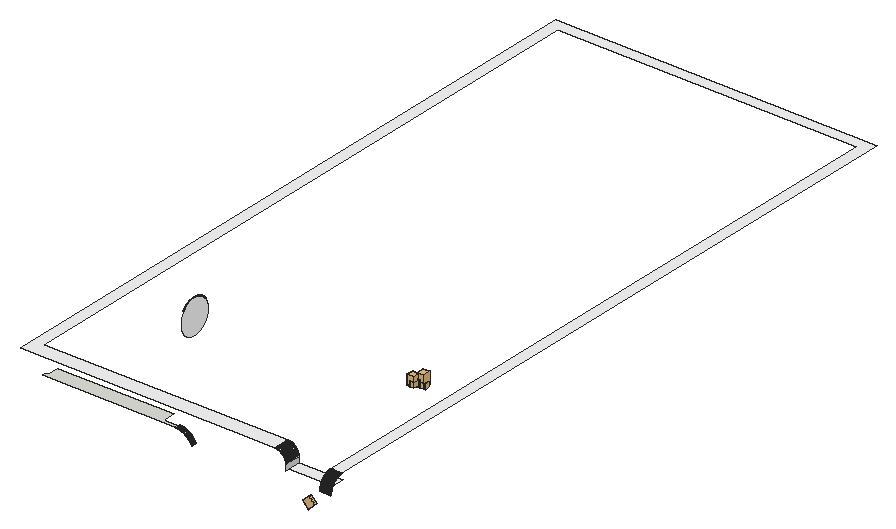
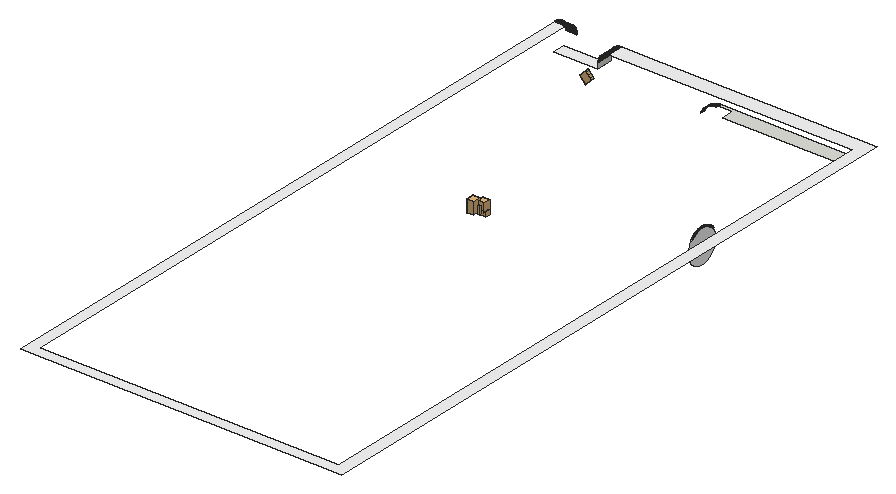
# SketchUp Ruby script. Lengths in inches.
U = 1.inch
M = Sketchup.active_model
def pt(a) = Geom::Point3d.new(a.map { |v| v * U })
def face(e, loops, mat)
  f = e.add_face(loops[0].map { |a| pt(a) })
  loops[1..].each { |l| e.add_face(l.map { |a| pt(a) }).erase! }
  f.material = f.back_material = mat if mat
  f
end
# faces: each face lists its corners as indices into pts; further lists are holes
def faces(e, pts, list, mat = nil) = list.each { |f| face(e, (f[0].is_a?(Array) ? f : [f]).map { |l| l.map { |i| pts[i] } }, mat) }
# xy, xz, yz: faces in a plane at the given z, y or x. An outline is a flat list of corners, or four numbers for a rectangle; further outlines are holes
def ring(l) = l.size == 4 ? [[l[0], l[1]], [l[2], l[1]], [l[2], l[3]], [l[0], l[3]]] : l.each_slice(2).to_a
def flat(e, list, mat, &to3) = list.each { |f| face(e, (f[0].is_a?(Array) ? f : [f]).map { |l| ring(l).map { |u, v| to3.(u, v) } }, mat) }
def xy(e, z, list, mat = nil) = flat(e, list, mat) { |x, y| [x, y, z] }
def xz(e, y, list, mat = nil) = flat(e, list, mat) { |x, z| [x, y, z] }
def yz(e, x, list, mat = nil) = flat(e, list, mat) { |y, z| [x, y, z] }
def lines(e, pts, list) = list.each { |a, b| e.add_line(pt(pts[a]), pt(pts[b])) }
# prism: a flat outline (further loops are holes) pulled along v
def prism(e, loops, v, mat = nil)
  f = face(e, loops, mat); d = Geom::Vector3d.new(v.map { |x| x * U })
  f.pushpull(f.normal.samedirection?(d) ? d.length : -d.length)
end
def box(e, o, s, mat = nil) = prism(e, [[o, [o[0] + s[0], o[1], o[2]], [o[0] + s[0], o[1] + s[1], o[2]], [o[0], o[1] + s[1], o[2]]]], [0, 0, s[2]], mat)
def at(x, y, z, deg = 0) = Geom::Transformation.translation(pt([x, y, z])) * Geom::Transformation.rotation(ORIGIN, Z_AXIS, deg.degrees)
def axes(o, x, y, z) = Geom::Transformation.new([*x, 0, *y, 0, *z, 0, *pt(o).to_a, 1])
def part(name) = M.definitions.add(name)
# library, detail: a bought-in or finely detailed component or shape, given as its bounding box
def library(name, o, s) = part(name).tap { |d| box(d.entities, o, s) }
def detail(e, o, s) = box(e.add_group.entities, o, s)
def put(e, d, t, mat = nil) = e.add_instance(d, t).tap { |i| i.material = mat if mat }
def group(e, t, mat = nil) = e.add_group.tap { |g| g.transformation = t; g.material = mat if mat }.entities
root = M.entities
M.materials.add("1448 AP 8253 RAVEN SONG").color = [0, 0, 0]
M.materials.add("[Quartz Light Grey]").color = [251, 251, 252]
c1 = library("Group\#187",[-292.81,-667.38,1418.14],[215.17,356.07,188.87])
c2 = library("Group\#181",[-278.4,-571.99,1530.91],[311.57,345.77,423.62])
c3 = library("Group\#168",[-264.68,-415.73,1484.11],[304.64,209.69,227.41])
c4 = library("Group\#175",[-357.04,-394.18,1447.05],[213.62,306.36,356.95])
c5 = library("Group\#182",[-548.25,-262.82,1459.54],[373.26,352.35,568])
c6 = library("Group\#184",[-387.74,-136.11,1470.07],[230,321.58,230.27])
c7 = library("Group\#22",[-1.75,-3,-1.85],[9.46,3.28,9.45])
xy(root,66,[[24,50,24,53,25.08,53,25.16,53.01,25.24,53.01,25.3125,53.02,25.39,53.04,25.47,53.06,25.54,53.08,25.62,53.1,25.69,53.125,25.77,53.15,25.84,53.18,25.98,53.26,26.04,53.29,26.11,53.34,26.18,53.38,26.36,53.53,26.41,53.59,26.47,53.64,26.62,53.82,26.66,53.89,26.71,53.96,26.74,54.02,26.82,54.16,26.85,54.23,26.875,54.31,26.9,54.38,26.92,54.46,26.94,54.53,26.96,54.61,26.98,54.6875,26.99,54.76,26.99,54.84,27,54.92,27,67,153,67,153,54.92,153.01,54.84,153.01,54.76,153.02,54.6875,153.04,54.61,153.06,54.53,153.08,54.46,153.1,54.38,153.125,54.31,153.15,54.23,153.18,54.16,153.26,54.02,153.29,53.96,153.34,53.89,153.38,53.82,153.53,53.64,153.59,53.59,153.64,53.53,153.82,53.38,153.89,53.34,153.96,53.29,154.02,53.26,154.16,53.18,154.23,53.15,154.31,53.125,154.38,53.1,154.46,53.08,154.53,53.06,154.61,53.04,154.6875,53.02,154.76,53.01,154.84,53.01,154.92,53,168,53,168,50],[168,50,168.29,53]])
xy(root,66,[[288,53.5,336,67]],"[Quartz Light Grey]")
xy(root,69,[[44.5,229.59,45,230.06]],"[Quartz Light Grey]")
xy(root,70,[[44.5,229.56,45,230.0625]],"[Quartz Light Grey]")
xy(root,83.99,[[336,50.41,348,50.61]],"[Quartz Light Grey]")
xy(root,84,[[0,50,257.5,50,257.5,50.25,258,50.25,258,50,276,50,276,67,12,67,12,763,336,763,336,51,348,51,348,775,0,775],[276,50,276.16,67],[276.16,50,276.3125,67],[336,50.8,348,51]],"[Quartz Light Grey]")
xz(root,36,[[336,69,348,69.2]],"[Quartz Light Grey]")
xz(root,36.01,[[336,69.39,348,69.59]],"[Quartz Light Grey]")
yz(root,45,[[229.94,33,230.41,33,230.88,33.02,231.35,33.05,231.82,33.09,232.76,33.21,233.22,33.29,233.69,33.38,234.14,33.48,235.06,33.72,235.51,33.86,235.95,34.01,236.4,34.17,236.83,34.35,237.27,34.53,237.7,34.73,238.54,35.15,238.95,35.38,239.35,35.62,239.75,35.87,240.15,36.13,240.53,36.4,240.91,36.68,241.28,36.97,241.65,37.27,242,37.58,242.35,37.9,242.6875,38.23,243.02,38.57,243.34,38.91,243.65,39.27,243.95,39.625,244.24,40,244.53,40.37,244.8,40.76,245.0625,41.15,245.32,41.55,245.56,41.95,245.79,42.36,246.01,42.78,246.22,43.2,246.42,43.625,246.61,44.06,246.78,44.49,246.95,44.9375,247.1,45.38,247.24,45.83,247.37,46.28,247.49,46.74,247.59,47.2,247.6875,47.66,247.77,48.125,247.84,48.59,247.9,49.06,247.94,49.53,247.97,50,247.99,50.47,248,50.94,248,51.41,247.98,51.88,247.95,52.35,247.91,52.82,247.79,53.76,247.71,54.22,247.62,54.69,247.52,55.14,247.28,56.06,247.14,56.51,246.99,56.95,246.83,57.4,246.65,57.83,246.47,58.27,246.27,58.7,245.85,59.54,245.62,59.95,245.38,60.35,245.13,60.75,244.87,61.15,244.6,61.53,244.32,61.91,244.03,62.28,243.73,62.65,243.42,63,243.1,63.35,242.77,63.6875,242.43,64.02,242.09,64.34,241.73,64.65,241.375,64.95,241,65.24,240.63,65.53,240.24,65.8,239.85,66.0625,239.45,66.32,239.05,66.56,238.64,66.79,238.22,67.01,237.8,67.22,237.375,67.42,236.94,67.61,236.51,67.78,236.0625,67.95,235.62,68.1,235.17,68.24,234.72,68.37,234.26,68.49,233.8,68.59,233.34,68.6875,232.875,68.77,232.41,68.84,231.94,68.9,231.47,68.94,231,68.97,230.53,68.99,230.06,69,229.59,69,229.12,68.98,228.65,68.95,228.18,68.91,227.24,68.79,226.78,68.71,226.31,68.62,225.86,68.52,224.94,68.28,224.49,68.14,224.05,67.99,223.6,67.83,223.17,67.65,222.73,67.47,222.3,67.27,221.46,66.85,221.05,66.62,220.65,66.38,220.25,66.13,219.85,65.87,219.47,65.6,219.09,65.32,218.72,65.03,218.35,64.73,218,64.42,217.65,64.1,217.3125,63.77,216.98,63.43,216.66,63.09,216.35,62.73,216.05,62.375,215.76,62,215.47,61.63,215.2,61.24,214.9375,60.85,214.68,60.45,214.44,60.05,214.21,59.64,213.99,59.22,213.78,58.8,213.58,58.375,213.39,57.94,213.22,57.51,213.05,57.0625,212.9,56.62,212.76,56.17,212.63,55.72,212.51,55.26,212.41,54.8,212.3125,54.34,212.23,53.875,212.16,53.41,212.1,52.94,212.06,52.47,212.03,52,212.01,51.53,212,51.06,212,50.59,212.02,50.12,212.05,49.65,212.09,49.18,212.21,48.24,212.29,47.78,212.38,47.31,212.48,46.86,212.72,45.94,212.86,45.49,213.01,45.05,213.17,44.6,213.35,44.17,213.53,43.73,213.73,43.3,214.15,42.46,214.38,42.05,214.62,41.65,214.87,41.25,215.13,40.85,215.4,40.47,215.68,40.09,215.97,39.72,216.27,39.35,216.58,39,216.9,38.65,217.23,38.3125,217.57,37.98,217.91,37.66,218.27,37.35,218.625,37.05,219,36.76,219.37,36.47,219.76,36.2,220.15,35.9375,220.55,35.68,220.95,35.44,221.36,35.21,221.78,34.99,222.2,34.78,222.625,34.58,223.06,34.39,223.49,34.22,223.9375,34.05,224.38,33.9,224.83,33.76,225.28,33.63,225.74,33.51,226.2,33.41,226.66,33.3125,227.125,33.23,227.59,33.16,228.06,33.1,228.53,33.06,229,33.03,229.47,33.01]],"[Quartz Light Grey]")
yz(root,288,[[50,66,67,72]])
yz(root,288,[[50,72,67,72.16],[50,72.16,67,72.3125]],"[Quartz Light Grey]")
p = [[185.89,55,54.26],[186,55,54],[186,50,54],[185.89,50,54.26],[185.77,55,54.53],[185.77,50,54.53],
  [185.65,55,54.79],[185.65,50,54.79],[185.53,55,55.04],[185.53,50,55.04],[185.4,55,55.3],[185.4,50,55.3],
  [185.27,55,55.56],[185.27,50,55.56],[185.13,55,55.81],[185.13,50,55.81],[185,55,56.06],[185,50,56.06],
  [184.85,55,56.31],[184.85,50,56.31],[184.71,55,56.56],[184.71,50,56.56],[184.56,55,56.8],[184.56,50,56.8],
  [184.4,55,57.04],[184.4,50,57.04],[184.25,55,57.28],[184.25,50,57.28],[184.09,55,57.52],[184.09,50,57.52],
  [183.92,55,57.76],[183.92,50,57.76],[183.76,55,57.99],[183.76,50,57.99],[183.59,55,58.22],[183.59,50,58.22],
  [183.41,55,58.45],[183.41,50,58.45],[183.23,55,58.67],[183.23,50,58.67],[183.05,55,58.89],[183.05,50,58.89],
  [182.87,55,59.11],[182.87,50,59.11],[182.68,55,59.33],[182.68,50,59.33],[182.49,55,59.55],[182.49,50,59.55],
  [182.3,55,59.76],[182.3,50,59.76],[182.1,55,59.97],[182.1,50,59.97],[181.9,55,60.17],[181.9,50,60.17],
  [181.7,55,60.375],[181.7,50,60.375],[181.5,55,60.58],[181.5,50,60.58],[181.29,55,60.77],[181.29,50,60.77],
  [181.08,55,60.97],[181.08,50,60.97],[180.86,55,61.16],[180.86,50,61.16],[180.65,55,61.34],[180.65,50,61.34],
  [180.43,55,61.53],[180.43,50,61.53],[180.2,55,61.71],[180.2,50,61.71],[179.98,55,61.89],[179.98,50,61.89],
  [179.75,55,62.0625],[179.75,50,62.0625],[179.52,55,62.23],[179.52,50,62.23],[179.29,55,62.4],[179.29,50,62.4],
  [179.05,55,62.5625],[179.05,50,62.5625],[178.82,55,62.72],[178.82,50,62.72],[45,215.27,63.01],[45,214.96,62.62],
  [44.5,214.96,62.62],[44.5,215.27,63.01],[45,243.42,63],[45,243.73,62.65],[44.5,243.73,62.65],[44.5,243.42,63],
  [178.58,55,62.88],[178.58,50,62.88],[45,216.35,62.73],[45,216.66,63.09],[44.5,216.66,63.09],[44.5,216.35,62.73],
  [178.34,55,63.04],[178.34,50,63.04],[45,244.8,62.91],[45,244.49,63.29],[44.5,244.49,63.29],[44.5,244.8,62.91],
  [178.09,55,63.1875],[178.09,50,63.1875],[45,215.59,63.39],[44.5,215.59,63.39],[45,243.1,63.35],[44.5,243.1,63.35],
  [45,216.98,63.43],[44.5,216.98,63.43],[177.84,55,63.33],[177.84,50,63.33],[177.6,55,63.48],[177.6,50,63.48],
  [45,242.77,63.6875],[44.5,242.77,63.6875],[45,244.16,63.67],[44.5,244.16,63.67],[45,215.92,63.76],[44.5,215.92,63.76],
  [45,217.3125,63.77],[44.5,217.3125,63.77],[177.35,55,63.61],[177.35,50,63.61],[177.09,55,63.75],[177.09,50,63.75],
  [45,242.43,64.02],[44.5,242.43,64.02],[45,243.82,64.03],[44.5,243.82,64.03],[176.84,55,63.88],[176.84,50,63.88],
  [45,216.26,64.125],[44.5,216.26,64.125],[45,217.65,64.1],[44.5,217.65,64.1],[176.58,55,64.01],[176.58,50,64.01],
  [176.32,55,64.13],[176.32,50,64.13],[45,242.09,64.34],[44.5,242.09,64.34],[45,243.48,64.39],[44.5,243.48,64.39],
  [176.0625,55,64.25],[176.0625,50,64.25],[45,216.61,64.48],[44.5,216.61,64.48],[45,218,64.42],[44.5,218,64.42],
  [175.8,55,64.37],[175.8,50,64.37],[45,241.73,64.65],[44.5,241.73,64.65],[175.54,55,64.48],[175.54,50,64.48],
  [45,218.35,64.73],[44.5,218.35,64.73],[45,243.125,64.74],[44.5,243.125,64.74],[175.27,55,64.59],[175.27,50,64.59],
  [45,216.97,64.82],[44.5,216.97,64.82],[175.01,55,64.7],[175.01,50,64.7],[45,241.375,64.95],[44.5,241.375,64.95],
  [174.74,55,64.8],[174.74,50,64.8],[45,218.72,65.03],[44.5,218.72,65.03],[45,242.76,65.08],[44.5,242.76,65.08],
  [174.47,55,64.9],[174.47,50,64.9],[45,217.33,65.16],[44.5,217.33,65.16],[174.2,55,64.99],[174.2,50,64.99],
  [173.92,55,65.08],[173.92,50,65.08],[45,219.09,65.32],[44.5,219.09,65.32],[45,241,65.24],[44.5,241,65.24],
  [173.65,55,65.16],[173.65,50,65.16],[45,242.39,65.41],[44.5,242.39,65.41],[173.1,55,65.32],[173.375,55,65.24],
  [173.375,50,65.24],[173.1,50,65.32],[45,217.71,65.49],[44.5,217.71,65.49],[45,240.63,65.53],[44.5,240.63,65.53],
  [172.82,55,65.39],[172.82,50,65.39],[45,219.47,65.6],[44.5,219.47,65.6],[172.54,55,65.46],[172.54,50,65.46],
  [45,242.01,65.73],[44.5,242.01,65.73],[171.98,55,65.59],[172.27,55,65.53],[172.27,50,65.53],[171.98,50,65.59],
  [45,218.09,65.8],[44.5,218.09,65.8],[45,240.24,65.8],[44.5,240.24,65.8],[171.42,55,65.7],[171.7,55,65.65],
  [171.7,50,65.65],[171.42,50,65.7],[45,219.85,65.87],[44.5,219.85,65.87],[170.86,55,65.79],[171.14,55,65.75],
  [171.14,50,65.75],[170.86,50,65.79],[45,241.62,66.04],[44.5,241.62,66.04],[170.29,55,65.87],[170.57,55,65.83],
  [170.57,50,65.83],[170.29,50,65.87],[45,218.48,66.11],[44.5,218.48,66.11],[45,239.85,66.0625],[44.5,239.85,66.0625],
  [169.15,55,65.97],[169.43,55,65.95],[169.43,50,65.95],[169.15,50,65.97],[169.72,55,65.92],[169.72,50,65.92],
  [170,55,65.9],[170,50,65.9],[45,220.25,66.13],[44.5,220.25,66.13],[168.29,50,66],[168.29,53,66],
  [168.57,53,65.99],[168.57,50,65.99],[168.86,53,65.98],[168.86,50,65.98],[169,53,65.97],[169,55,65.97],
  [45,241.22,66.33],[44.5,241.22,66.33],[45,218.88,66.41],[44.5,218.88,66.41],[45,220.65,66.38],[44.5,220.65,66.38],
  [45,239.45,66.32],[44.5,239.45,66.32],[45,239.05,66.56],[44.5,239.05,66.56],[45,240.8125,66.625],[44.5,240.8125,66.625],
  [45,219.29,66.69],[44.5,219.29,66.69],[45,221.05,66.62],[44.5,221.05,66.62],[45,221.46,66.85],[44.5,221.46,66.85],
  [45,238.64,66.79],[44.5,238.64,66.79],[45,240.4,66.9],[44.5,240.4,66.9],[45,219.7,66.97],[44.5,219.7,66.97],
  [45,221.88,67.06],[44.5,221.88,67.06],[45,238.22,67.01],[44.5,238.22,67.01],[45,239.98,67.17],[44.5,239.98,67.17],
  [45,220.125,67.23],[44.5,220.125,67.23],[45,237.8,67.22],[44.5,237.8,67.22],[45,222.3,67.27],[44.5,222.3,67.27],
  [45,220.55,67.49],[44.5,220.55,67.49],[45,237.375,67.42],[44.5,237.375,67.42],[45,239.55,67.42],[44.5,239.55,67.42],
  [45,222.73,67.47],[44.5,222.73,67.47],[45,236.94,67.61],[44.5,236.94,67.61],[45,239.12,67.67],[44.5,239.12,67.67],
  [45,220.99,67.73],[44.5,220.99,67.73],[45,223.17,67.65],[44.5,223.17,67.65],[45,236.51,67.78],[44.5,236.51,67.78],
  [45,221.43,67.96],[44.5,221.43,67.96],[45,223.6,67.83],[44.5,223.6,67.83],[45,238.68,67.9],[44.5,238.68,67.9],
  [45,224.05,67.99],[44.5,224.05,67.99],[45,236.0625,67.95],[44.5,236.0625,67.95],[45,235.62,68.1],[44.5,235.62,68.1],
  [45,238.24,68.12],[44.5,238.24,68.12],[45,221.875,68.18],[44.5,221.875,68.18],[45,224.49,68.14],[44.5,224.49,68.14],
  [45,224.94,68.28],[44.5,224.94,68.28],[45,235.17,68.24],[44.5,235.17,68.24],[45,237.78,68.33],[44.5,237.78,68.33],
  [45,222.33,68.38],[44.5,222.33,68.38],[45,234.72,68.37],[44.5,234.72,68.37],[45,225.4,68.4],[44.5,225.4,68.4],
  [45,237.33,68.53],[44.5,237.33,68.53],[45,222.79,68.58],[44.5,222.79,68.58],[45,225.86,68.52],[44.5,225.86,68.52],
  [45,234.26,68.49],[44.5,234.26,68.49],[45,226.31,68.62],[44.5,226.31,68.62],[45,233.8,68.59],[44.5,233.8,68.59],
  [45,236.87,68.72],[44.5,236.87,68.72],[45,223.25,68.76],[44.5,223.25,68.76],[45,226.78,68.71],[44.5,226.78,68.71],
  [45,233.34,68.6875],[44.5,233.34,68.6875],[45,227.24,68.79],[44.5,227.24,68.79],[45,232.875,68.77],[44.5,232.875,68.77],
  [45,236.4,68.89],[44.5,236.4,68.89],[45,223.72,68.93],[44.5,223.72,68.93],[45,227.71,68.85],[44.5,227.71,68.85],
  [45,231.94,68.9],[45,232.41,68.84],[44.5,232.41,68.84],[44.5,231.94,68.9],[45,224.1875,69.09],[44.5,224.1875,69.09],
  [45,228.18,68.91],[44.5,228.18,68.91],[45,228.65,68.95],[44.5,228.65,68.95],[45,229.12,68.98],[44.5,229.12,68.98],
  [45,231,68.97],[45,231.47,68.94],[44.5,231.47,68.94],[44.5,231,68.97],[45,235.93,69.05],[44.5,235.93,69.05],
  [45,229.59,69],[44.5,229.59,69],[45,230.06,69],[45,230.53,68.99],[44.5,230.53,68.99],[44.5,230.06,69],
  [45,224.66,69.24],[44.5,224.66,69.24],[45,235.46,69.2],[44.5,235.46,69.2],[336,36.01,69.39],[336,36,69.2],
  [348,36,69.2],[348,36.01,69.39],[45,225.14,69.37],[44.5,225.14,69.37],[45,234.98,69.34],[44.5,234.98,69.34],
  [45,234.5,69.46],[44.5,234.5,69.46],[45,225.625,69.49],[44.5,225.625,69.49],[45,226.11,69.6],[44.5,226.11,69.6],
  [45,234.01,69.57],[44.5,234.01,69.57],[336,36.02,69.79],[336,36.01,69.59],[348,36.01,69.59],[348,36.02,69.79],
  [45,226.6,69.69],[44.5,226.6,69.69],[45,233.52,69.67],[44.5,233.52,69.67],[45,227.09,69.78],[44.5,227.09,69.78],
  [45,233.03,69.76],[44.5,233.03,69.76],[336,36.03,69.98],[348,36.03,69.98],[45,227.58,69.85],[44.5,227.58,69.85],
  [45,228.08,69.9],[44.5,228.08,69.9],[45,232.54,69.83],[45,232.05,69.89],[44.5,232.05,69.89],[44.5,232.54,69.83],
  [45,228.57,69.95],[44.5,228.57,69.95],[45,229.07,69.98],[44.5,229.07,69.98],[45,231.55,69.9375],[45,231.06,69.97],
  [44.5,231.06,69.97],[44.5,231.55,69.9375],[336,36.05,70.18],[348,36.03,70],[348,36.05,70.18],[45,229.56,70],
  [44.5,229.56,70],[45,230.56,69.99],[45,230.0625,70],[44.5,230.0625,70],[44.5,230.56,69.99],[336,36.0625,70.37],
  [348,36.0625,70.37],[336,36.08,70.57],[348,36.08,70.57],[336,36.1,70.76],[348,36.1,70.76],[336,36.13,70.96],
  [348,36.13,70.96],[336,36.16,71.15],[348,36.16,71.15],[336,36.18,71.35],[348,36.18,71.35],[336,36.22,71.54],
  [348,36.22,71.54],[336,36.25,71.73],[348,36.25,71.73],[336,36.29,71.93],[348,36.29,71.93],[336,36.33,72.12],
  [348,36.33,72.12],[336,36.37,72.31],[348,36.37,72.31],[336,36.41,72.5],[348,36.41,72.5],[287.99,67,72.47],
  [287.99,50,72.47],[288,50,72.3125],[288,67,72.3125],[336,36.46,72.69],[348,36.46,72.69],[287.98,67,72.63],
  [287.98,50,72.63],[287.97,67,72.78],[287.97,50,72.78],[336,36.51,72.88],[348,36.51,72.88],[287.96,67,72.94],
  [287.96,50,72.94],[336,36.5625,73.07],[348,36.5625,73.07],[287.95,67,73.1],[287.95,50,73.1],[336,36.62,73.26],
  [348,36.62,73.26],[287.93,67,73.25],[287.93,50,73.25],[336,36.67,73.45],[348,36.67,73.45],[287.92,67,73.41],
  [287.92,50,73.41],[336,36.73,73.64],[348,36.73,73.64],[287.9,67,73.57],[287.9,50,73.57],[336,36.8,73.82],
  [348,36.8,73.82],[287.875,67,73.72],[287.875,50,73.72],[287.85,67,73.88],[287.85,50,73.88],[336,36.86,74.01],
  [348,36.86,74.01],[287.83,67,74.03],[287.83,50,74.03],[336,36.93,74.19],[348,36.93,74.19],[287.8,67,74.1875],
  [287.8,50,74.1875],[336,37,74.375],[348,37,74.375],[287.77,67,74.34],[287.77,50,74.34],[287.74,67,74.49],
  [287.74,50,74.49],[336,37.07,74.56],[348,37.07,74.56],[287.7,67,74.65],[287.7,50,74.65],[336,37.14,74.74],
  [348,37.14,74.74],[287.67,67,74.8],[287.67,50,74.8],[336,37.22,74.92],[348,37.22,74.92],[287.63,67,74.95],
  [287.63,50,74.95],[336,37.3,75.1],[348,37.3,75.1],[287.59,67,75.11],[287.59,50,75.11],[336,37.38,75.28],
  [348,37.38,75.28],[287.55,67,75.26],[287.55,50,75.26],[336,37.46,75.46],[348,37.46,75.46],[287.51,67,75.41],
  [287.51,50,75.41],[287.46,67,75.56],[287.46,50,75.56],[336,37.55,75.63],[348,37.55,75.63],[336,37.63,75.81],
  [348,37.63,75.81],[287.41,67,75.71],[287.41,50,75.71],[287.36,67,75.86],[287.36,50,75.86],[336,37.73,75.98],
  [348,37.73,75.98],[287.3125,67,76.01],[287.3125,50,76.01],[336,37.82,76.16],[348,37.82,76.16],[287.26,67,76.15],
  [287.26,50,76.15],[336,37.91,76.33],[348,37.91,76.33],[287.2,67,76.3],[287.2,50,76.3],[336,38.01,76.5],
  [348,38.01,76.5],[287.15,67,76.45],[287.15,50,76.45],[287.09,67,76.59],[287.09,50,76.59],[336,38.11,76.67],
  [348,38.11,76.67],[287.03,67,76.74],[287.03,50,76.74],[336,38.21,76.84],[348,38.21,76.84],[286.96,67,76.88],
  [286.96,50,76.88],[336,38.3125,77],[348,38.3125,77],[286.9,67,77.02],[286.9,50,77.02],[336,38.42,77.17],
  [348,38.42,77.17],[286.83,67,77.17],[286.83,50,77.17],[336,38.53,77.33],[348,38.53,77.33],[286.76,67,77.31],
  [286.76,50,77.31],[336,38.64,77.5],[348,38.64,77.5],[286.69,67,77.45],[286.69,50,77.45],[286.62,67,77.59],
  [286.62,50,77.59],[336,38.75,77.66],[348,38.75,77.66],[286.55,67,77.73],[286.55,50,77.73],[336,38.86,77.82],
  [348,38.86,77.82],[286.47,67,77.86],[286.47,50,77.86],[336,38.98,77.97],[348,38.98,77.97],[286.39,67,78],
  [286.39,50,78],[336,39.1,78.13],[348,39.1,78.13],[286.3125,67,78.14],[286.3125,50,78.14],[336,39.22,78.29],
  [348,39.22,78.29],[286.23,67,78.27],[286.23,50,78.27],[336,39.34,78.44],[348,39.34,78.44],[286.15,67,78.4],
  [286.15,50,78.4],[336,39.47,78.59],[348,39.47,78.59],[286.0625,67,78.54],[286.0625,50,78.54],[285.98,67,78.67],
  [285.98,50,78.67],[336,39.59,78.74],[348,39.59,78.74],[336,39.72,78.89],[348,39.72,78.89],[285.89,67,78.8],
  [285.89,50,78.8],[285.8,67,78.93],[285.8,50,78.93],[336,39.85,79.04],[348,39.85,79.04],[285.71,67,79.05],
  [285.71,50,79.05],[336,39.99,79.18],[348,39.99,79.18],[285.62,67,79.18],[285.62,50,79.18],[336,40.12,79.33],
  [348,40.12,79.33],[285.52,67,79.31],[285.52,50,79.31],[336,40.26,79.47],[348,40.26,79.47],[285.42,67,79.43],
  [285.42,50,79.43],[285.33,67,79.55],[285.33,50,79.55],[336,40.39,79.61],[348,40.39,79.61],[336,40.53,79.74],
  [348,40.53,79.74],[285.23,67,79.67],[285.23,50,79.67],[336,40.67,79.88],[348,40.67,79.88],[285.125,67,79.79],
  [285.125,50,79.79],[285.02,67,79.91],[285.02,50,79.91],[336,40.82,80.01],[348,40.82,80.01],[284.92,67,80.03],
  [284.92,50,80.03],[336,40.96,80.15],[348,40.96,80.15],[284.8125,67,80.15],[284.8125,50,80.15],[336,41.11,80.28],
  [348,41.11,80.28],[284.7,67,80.26],[284.7,50,80.26],[336,41.26,80.41],[348,41.26,80.41],[284.6,67,80.375],
  [284.6,50,80.375],[336,41.41,80.53],[348,41.41,80.53],[284.49,67,80.49],[284.49,50,80.49],[336,41.56,80.66],
  [348,41.56,80.66],[284.375,67,80.6],[284.375,50,80.6],[284.26,67,80.7],[284.26,50,80.7],[336,41.71,80.78],
  [348,41.71,80.78],[284.15,67,80.8125],[284.15,50,80.8125],[336,41.87,80.9],[348,41.87,80.9],[284.03,67,80.92],
  [284.03,50,80.92],[336,42.03,81.02],[348,42.03,81.02],[283.91,67,81.02],[283.91,50,81.02],[336,42.18,81.14],
  [348,42.18,81.14],[283.79,67,81.125],[283.79,50,81.125],[336,42.34,81.25],[348,42.34,81.25],[283.67,67,81.23],
  [283.67,50,81.23],[336,42.5,81.36],[348,42.5,81.36],[283.55,67,81.33],[283.55,50,81.33],[283.43,67,81.42],
  [283.43,50,81.42],[336,42.67,81.47],[348,42.67,81.47],[283.31,67,81.52],[283.31,50,81.52],[336,42.83,81.58],
  [348,42.83,81.58],[283.18,67,81.62],[283.18,50,81.62],[336,43,81.6875],[348,43,81.6875],[283.05,67,81.71],
  [283.05,50,81.71],[336,43.16,81.79],[348,43.16,81.79],[282.93,67,81.8],[282.93,50,81.8],[336,43.33,81.89],
  [348,43.33,81.89],[282.8,67,81.89],[282.8,50,81.89],[336,43.5,81.99],[348,43.5,81.99],[282.67,67,81.98],
  [282.67,50,81.98],[336,43.67,82.09],[348,43.67,82.09],[282.54,67,82.0625],[282.54,50,82.0625],[336,43.84,82.18],
  [348,43.84,82.18],[282.27,67,82.23],[282.27,50,82.23],[282.4,50,82.15],[282.4,67,82.15],[336,44.02,82.27],
  [348,44.02,82.27],[282.14,67,82.3125],[282.14,50,82.3125],[336,44.19,82.37],[348,44.19,82.37],[282,67,82.39],
  [282,50,82.39],[336,44.37,82.45],[348,44.37,82.45],[281.86,67,82.47],[281.86,50,82.47],[336,44.54,82.54],
  [348,44.54,82.54],[336,44.72,82.62],[348,44.72,82.62],[281.59,67,82.62],[281.59,50,82.62],[281.73,50,82.55],
  [281.73,67,82.55],[336,44.9,82.7],[348,44.9,82.7],[281.45,67,82.69],[281.45,50,82.69],[336,45.08,82.78],
  [348,45.08,82.78],[281.31,67,82.76],[281.31,50,82.76],[336,45.26,82.86],[348,45.26,82.86],[281.02,67,82.9],
  [281.02,50,82.9],[281.17,50,82.83],[281.17,67,82.83],[336,45.44,82.93],[348,45.44,82.93],[336,45.625,83],
  [348,45.625,83],[280.88,67,82.96],[280.88,50,82.96],[336,45.81,83.07],[348,45.81,83.07],[280.59,67,83.09],
  [280.59,50,83.09],[280.74,50,83.03],[280.74,67,83.03],[336,45.99,83.14],[348,45.99,83.14],[336,46.18,83.2],
  [348,46.18,83.2],[280.3,67,83.2],[280.3,50,83.2],[280.45,50,83.15],[280.45,67,83.15],[336,46.36,83.27],
  [348,46.36,83.27],[280.15,67,83.26],[280.15,50,83.26],[336,46.55,83.33],[348,46.55,83.33],[336,46.74,83.38],
  [348,46.74,83.38],[279.86,67,83.36],[279.86,50,83.36],[280.01,50,83.3125],[280.01,67,83.3125],[336,46.93,83.4375],
  [348,46.93,83.4375],[336,47.12,83.49],[348,47.12,83.49],[279.56,67,83.46],[279.56,50,83.46],[279.71,50,83.41],
  [279.71,67,83.41],[336,47.31,83.54],[348,47.31,83.54],[336,47.5,83.59],[348,47.5,83.59],[279.11,67,83.59],
  [279.11,50,83.59],[279.26,50,83.55],[279.26,67,83.55],[279.41,50,83.51],[279.41,67,83.51],[336,47.69,83.63],
  [348,47.69,83.63],[336,47.88,83.67],[348,47.88,83.67],[278.8,67,83.67],[278.8,50,83.67],[278.95,50,83.63],
  [278.95,67,83.63],[336,48.07,83.71],[348,48.07,83.71],[336,48.27,83.75],[348,48.27,83.75],[336,48.46,83.78],
  [348,48.46,83.78],[278.34,67,83.77],[278.34,50,83.77],[278.49,50,83.74],[278.49,67,83.74],[278.65,50,83.7],
  [278.65,67,83.7],[336,48.65,83.82],[348,48.65,83.82],[336,48.85,83.84],[348,48.85,83.84],[336,49.04,83.87],
  [348,49.04,83.87],[277.88,67,83.85],[277.88,50,83.85],[278.03,50,83.83],[278.03,67,83.83],[278.1875,50,83.8],
  [278.1875,67,83.8],[336,49.24,83.9],[348,49.24,83.9],[336,49.43,83.92],[348,49.43,83.92],[336,49.63,83.9375],
  [348,49.63,83.9375],[336,49.82,83.95],[348,49.82,83.95],[276.94,67,83.96],[276.94,50,83.96],[277.1,50,83.95],
  [277.1,67,83.95],[277.25,50,83.93],[277.25,67,83.93],[277.41,50,83.92],[277.41,67,83.92],[277.57,50,83.9],
  [277.57,67,83.9],[277.72,50,83.875],[277.72,67,83.875],[336,50.02,83.97],[348,50.02,83.97],[276.3125,67,84],
  [276.3125,50,84],[276.47,50,83.99],[276.47,67,83.99],[276.63,50,83.98],[276.63,67,83.98],[276.78,50,83.97],
  [276.78,67,83.97],[336,50.21,83.98],[348,50.21,83.98],[336,50.41,83.99],[348,50.41,83.99],[336,50.8,84],
  [336,50.61,83.99],[348,50.61,83.99],[348,50.8,84],[169,55,66]]
faces(root,p,[[0,1,2,3],[4,0,3,5],[6,4,5,7],[8,6,7,9],[10,8,9,11],[12,10,11,13],[14,12,13,15],[16,14,15,17],
  [18,16,17,19],[20,18,19,21],[22,20,21,23],[24,22,23,25],[26,24,25,27],[28,26,27,29],[30,28,29,31],[32,30,31,33],
  [34,32,33,35],[36,34,35,37],[38,36,37,39],[40,38,39,41],[42,40,41,43],[44,42,43,45],[46,44,45,47],[48,46,47,49],
  [50,48,49,51],[52,50,51,53],[54,52,53,55],[56,54,55,57],[58,56,57,59],[60,58,59,61],[62,60,61,63],[64,62,63,65],
  [66,64,65,67],[68,66,67,69],[70,68,69,71],[72,70,71,73],[74,72,73,75],[76,74,75,77],[78,76,77,79],[80,78,79,81],
  [90,80,81,91],[96,90,91,97],[102,96,97,103],[110,102,103,111],[112,110,111,113],[122,112,113,123],[124,122,123,125],[130,124,125,131],
  [136,130,131,137],[138,136,137,139],[144,138,139,145],[150,144,145,151],[154,150,151,155],[160,154,155,161],[164,160,161,165],[168,164,165,169],
  [174,168,169,175],[178,174,175,179],[180,178,179,181],[186,180,181,187],[190,191,192,193],[191,186,187,192],[198,190,193,199],[202,198,199,203],
  [206,207,208,209],[207,202,203,208],[214,215,216,217],[215,206,209,216],[220,221,222,223],[221,214,217,222],[226,227,228,229],[227,220,223,228],
  [234,235,236,237],[235,238,239,236],[238,240,241,239],[240,226,229,241],[244,245,246,247],[247,246,248,249],[249,248,250,251,234,237]])
faces(root,p,[[82,83,84,85],[86,87,88,89],[92,93,94,95],[98,99,100,101],[104,82,85,105],[106,86,89,107],[93,108,109,94],[114,106,107,115],
  [99,116,117,100],[118,104,105,119],[108,120,121,109],[126,114,115,127],[116,128,129,117],[132,118,119,133],[120,134,135,121],[140,126,127,141],
  [128,142,143,129],[146,132,133,147],[134,148,149,135],[152,140,141,153],[148,156,157,149],[142,158,159,143],[162,146,147,163],[166,152,153,167],
  [156,170,171,157],[158,172,173,159],[176,162,163,177],[170,182,183,171],[184,166,167,185],[172,188,189,173],[194,176,177,195],[196,184,185,197],
  [182,200,201,183],[188,204,205,189],[210,194,195,211],[212,196,197,213],[200,218,219,201],[204,224,225,205],[230,210,211,231],[232,212,213,233],
  [218,242,243,219],[224,252,253,225],[254,230,231,255],[242,256,257,243],[258,232,233,259],[260,258,259,261],[252,262,263,253],[264,254,255,265],
  [256,266,267,257],[266,268,269,267],[270,260,261,271],[262,272,273,263],[274,264,265,275],[268,276,277,269],[278,270,271,279],[272,280,281,273],
  [282,274,275,283],[284,278,279,285],[276,286,287,277],[288,282,283,289],[290,284,285,291],[280,292,293,281],[286,294,295,287],[296,290,291,297],
  [292,298,299,293],[300,288,289,301],[294,302,303,295],[304,296,297,305],[306,300,301,307],[302,308,309,303],[298,310,311,299],[308,312,313,309],
  [314,304,305,315],[316,314,315,317],[310,318,319,311],[320,306,307,321],[312,322,323,313],[322,324,325,323],[326,316,317,327],[318,328,329,319],
  [330,320,321,331],[332,326,327,333],[324,334,335,325],[328,336,337,329],[338,330,331,339],[334,340,341,335],[342,332,333,343],[340,344,345,341],
  [346,342,343,347],[336,348,349,337],[350,338,339,351],[344,352,353,345],[354,346,347,355],[352,356,357,353],[358,354,355,359],[348,360,361,349],
  [362,350,351,363],[356,364,365,357],[366,367,368,369],[367,358,359,368],[370,362,363,371],[364,372,373,365],[372,374,375,373],[374,376,377,375],
  [378,379,380,381],[379,366,369,380],[360,382,383,361],[376,384,385,377],[386,387,388,389],[387,378,381,388],[390,370,371,391],[382,392,393,383],
  [394,395,396,397],[398,390,391,399],[392,400,401,393],[400,402,403,401],[404,398,399,405],[406,404,405,407],[402,408,409,403],[410,411,412,413],
  [414,406,407,415],[408,416,417,409],[418,414,415,419],[416,420,421,417],[422,410,413,423],[424,418,419,425],[426,424,425,427],[428,429,430,431],
  [420,428,431,421],[432,426,427,433],[434,432,433,435],[436,437,438,439],[429,436,439,430],[440,422,423,441,442],[443,434,435,444],[445,446,447,448],
  [437,445,448,438],[449,440,442,450],[451,449,450,452],[453,451,452,454],[455,453,454,456],[457,455,456,458],[459,457,458,460],[461,459,460,462],
  [463,461,462,464],[465,463,464,466],[467,465,466,468],[469,467,468,470],[471,469,470,472],[473,474,475,476],[477,471,472,478],[479,480,474,473],
  [481,482,480,479],[483,477,478,484],[485,486,482,481],[487,483,484,488],[489,490,486,485],[491,487,488,492],[493,494,490,489],[495,491,492,496],
  [497,498,494,493],[499,495,496,500],[501,502,498,497],[503,499,500,504],[505,506,502,501],[507,508,506,505],[509,503,504,510],[511,512,508,507],
  [513,509,510,514],[515,516,512,511],[517,513,514,518],[519,520,516,515],[521,522,520,519],[523,517,518,524],[525,526,522,521],[527,523,524,528],
  [529,530,526,525],[531,527,528,532],[533,534,530,529],[535,531,532,536],[537,538,534,533],[539,535,536,540],[541,542,538,537],[543,539,540,544],
  [545,546,542,541],[547,548,546,545],[549,543,544,550],[551,549,550,552],[553,554,548,547],[555,556,554,553],[557,551,552,558],[559,560,556,555],
  [561,557,558,562],[563,564,560,559],[565,561,562,566],[567,568,564,563],[569,565,566,570],[571,572,568,567],[573,574,572,571],[575,569,570,576],
  [577,578,574,573],[579,575,576,580],[581,582,578,577],[583,579,580,584],[585,586,582,581],[587,583,584,588],[589,590,586,585],[591,587,588,592],
  [593,594,590,589],[595,591,592,596],[597,598,594,593],[599,600,598,597],[601,595,596,602],[603,604,600,599],[605,601,602,606],[607,608,604,603],
  [609,605,606,610],[611,612,608,607],[613,609,610,614],[615,616,612,611],[617,613,614,618],[619,620,616,615],[621,617,618,622],[623,624,620,619],
  [625,621,622,626],[627,628,624,623],[629,630,628,627],[631,625,626,632],[633,631,632,634],[635,636,630,629],[637,638,636,635],[639,633,634,640],
  [641,642,638,637],[643,639,640,644],[645,646,642,641],[647,643,644,648],[649,650,646,645],[651,647,648,652],[653,654,650,649],[655,656,654,653],
  [657,651,652,658],[659,657,658,660],[661,662,656,655],[663,659,660,664],[665,666,662,661],[667,668,666,665],[669,663,664,670],[671,672,668,667],
  [673,669,670,674],[675,676,672,671],[677,673,674,678],[679,680,676,675],[681,677,678,682],[683,684,680,679],[685,681,682,686],[687,688,684,683],
  [689,685,686,690],[691,692,688,687],[693,694,692,691],[695,689,690,696],[697,698,694,693],[699,695,696,700],[701,702,698,697],[703,699,700,704],
  [705,706,702,701],[707,703,704,708],[709,710,706,705],[711,707,708,712],[713,714,710,709],[715,711,712,716],[717,718,714,713],[719,720,718,717],
  [721,715,716,722],[723,724,720,719],[725,721,722,726],[727,728,724,723],[729,725,726,730],[731,732,728,727],[733,729,730,734],[735,736,732,731],
  [737,733,734,738],[739,740,736,735],[741,737,738,742],[743,744,740,739],[745,741,742,746],[747,748,744,743],[749,745,746,750],[751,752,753,754],
  [754,753,748,747],[755,749,750,756],[757,758,752,751],[759,755,756,760],[761,762,758,757],[763,759,760,764],[765,766,762,761],[767,763,764,768],
  [769,767,768,770],[771,772,773,774],[774,773,766,765],[775,769,770,776],[777,778,772,771],[779,775,776,780],[781,782,778,777],[783,779,780,784],
  [785,786,787,788],[788,787,782,781],[789,783,784,790],[791,789,790,792],[793,794,786,785],[795,791,792,796],[797,798,799,800],[800,799,794,793],
  [801,795,796,802],[803,801,802,804],[805,806,807,808],[808,807,798,797],[809,803,804,810],[811,812,806,805],[813,809,810,814],[815,813,814,816],
  [817,818,819,820],[820,819,812,811],[821,815,816,822],[823,821,822,824],[825,826,827,828],[828,827,818,817],[829,823,824,830],[831,829,830,832],
  [833,834,835,836],[836,835,837,838],[838,837,826,825],[839,831,832,840],[841,839,840,842],[843,844,845,846],[846,845,834,833],[847,841,842,848],
  [849,847,848,850],[851,849,850,852],[853,854,855,856],[856,855,857,858],[858,857,844,843],[859,851,852,860],[861,859,860,862],[863,861,862,864],
  [865,866,867,868],[868,867,869,870],[870,869,854,853],[871,863,864,872],[873,871,872,874],[875,873,874,876],[877,875,876,878],[879,880,881,882],
  [882,881,883,884],[884,883,885,886],[886,885,887,888],[888,887,889,890],[890,889,866,865],[891,877,878,892],[893,894,895,896],[896,895,897,898],
  [898,897,899,900],[900,899,880,879],[901,891,892,902],[903,901,902,904],[905,906,907,908]],"[Quartz Light Grey]")
lines(root,p,[[909,251]])
put(root,c1,axes([253.68,273.14,0.11],[0,-0.02318,0],[0.02157,0,0],[0,0,0.02333]))
put(root,c2,axes([253.68,273.14,0.11],[0,-0.02318,0],[0.02157,0,0],[0,0,0.02333]))
put(root,c3,axes([253.68,273.14,0.11],[0,-0.02318,0],[0.02157,0,0],[0,0,0.02333]))
put(root,c4,axes([253.68,273.14,0.11],[0,-0.02318,0],[0.02157,0,0],[0,0,0.02333]))
put(root,c5,axes([253.68,273.14,0.11],[0,-0.02318,0],[0.02157,0,0],[0,0,0.02333]))
put(root,c6,axes([253.68,273.14,0.11],[0,-0.02318,0],[0.02157,0,0],[0,0,0.02333]))
put(root,c7,axes([312.17,53.22,38.95],[0.70711,0,0.70711],[0,1,0],[-0.70711,0,0.70711]),"1448 AP 8253 RAVEN SONG")
